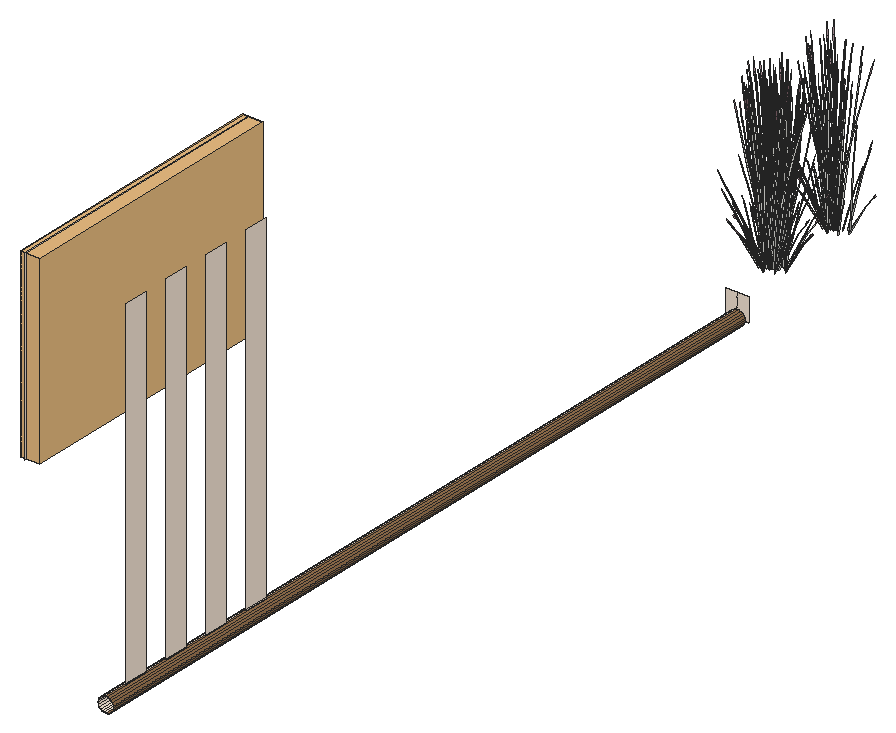
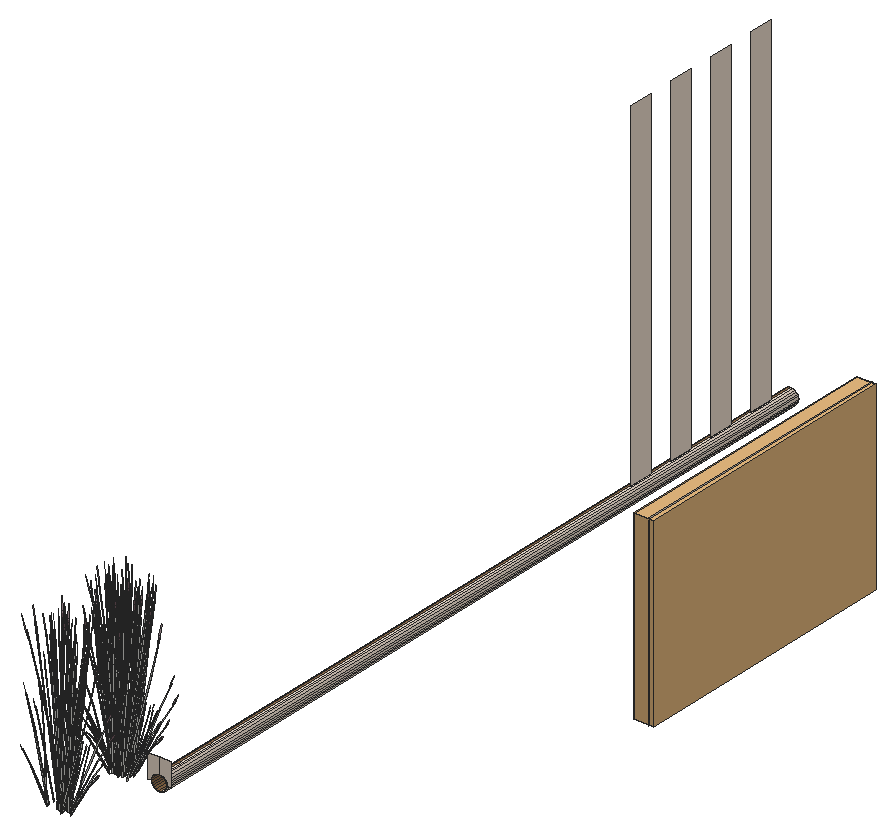
# SketchUp Ruby script. Lengths in inches.
U = 1.inch
M = Sketchup.active_model
def pt(a) = Geom::Point3d.new(a.map { |v| v * U })
def face(e, loops, mat)
  f = e.add_face(loops[0].map { |a| pt(a) })
  loops[1..].each { |l| e.add_face(l.map { |a| pt(a) }).erase! }
  f.material = f.back_material = mat if mat
  f
end
# faces: each face lists its corners as indices into pts; further lists are holes
def faces(e, pts, list, mat = nil) = list.each { |f| face(e, (f[0].is_a?(Array) ? f : [f]).map { |l| l.map { |i| pts[i] } }, mat) }
# xy, xz, yz: faces in a plane at the given z, y or x. An outline is a flat list of corners, or four numbers for a rectangle; further outlines are holes
def ring(l) = l.size == 4 ? [[l[0], l[1]], [l[2], l[1]], [l[2], l[3]], [l[0], l[3]]] : l.each_slice(2).to_a
def flat(e, list, mat, &to3) = list.each { |f| face(e, (f[0].is_a?(Array) ? f : [f]).map { |l| ring(l).map { |u, v| to3.(u, v) } }, mat) }
def xy(e, z, list, mat = nil) = flat(e, list, mat) { |x, y| [x, y, z] }
def xz(e, y, list, mat = nil) = flat(e, list, mat) { |x, z| [x, y, z] }
def yz(e, x, list, mat = nil) = flat(e, list, mat) { |y, z| [x, y, z] }
def lines(e, pts, list) = list.each { |a, b| e.add_line(pt(pts[a]), pt(pts[b])) }
# prism: a flat outline (further loops are holes) pulled along v
def prism(e, loops, v, mat = nil)
  f = face(e, loops, mat); d = Geom::Vector3d.new(v.map { |x| x * U })
  f.pushpull(f.normal.samedirection?(d) ? d.length : -d.length)
end
def box(e, o, s, mat = nil) = prism(e, [[o, [o[0] + s[0], o[1], o[2]], [o[0] + s[0], o[1] + s[1], o[2]], [o[0], o[1] + s[1], o[2]]]], [0, 0, s[2]], mat)
def at(x, y, z, deg = 0) = Geom::Transformation.translation(pt([x, y, z])) * Geom::Transformation.rotation(ORIGIN, Z_AXIS, deg.degrees)
def axes(o, x, y, z) = Geom::Transformation.new([*x, 0, *y, 0, *z, 0, *pt(o).to_a, 1])
def part(name) = M.definitions.add(name)
# library, detail: a bought-in or finely detailed component or shape, given as its bounding box
def library(name, o, s) = part(name).tap { |d| box(d.entities, o, s) }
def detail(e, o, s) = box(e.add_group.entities, o, s)
def put(e, d, t, mat = nil) = e.add_instance(d, t).tap { |i| i.material = mat if mat }
def group(e, t, mat = nil) = e.add_group.tap { |g| g.transformation = t; g.material = mat if mat }.entities
root = M.entities
M.materials.add("C01_Vanilla_Cream").color = [244, 228, 212]
M.materials.add("LightPink_Translucent").color = [144, 107, 117]
M.materials["LightPink_Translucent"].alpha = 0.75
M.materials.add("Wood_Floor_01_1K").color = [146, 111, 76]
c1 = library("Double casement window",[0,0,0],[5.02,56.42,60])
c2 = part("blade")
p = [[2.15,0.21,22],[0,0.17,0],[0.09,0.45,0],[2.18,0.31,22],[2.29,0.31,22],[0.38,0.45,0],
  [2.48,0.24,33],[2.49,0.24,33],[2.48,0.22,33]]
faces(c2.entities,p,[[0,1,2,3],[4,5,2,3],[6,3,4,7],[8,0,3,6]])
c3 = part("seeds")
p = [[0.3,-0.1,1.38],[-0.01,-0.03,1.59],[-0.01,-0.03,0.03],[0.14,-0.07,-0.07],[0.29,-0.03,3],[0.15,0.01,3.11]]
faces(c3.entities,p,[[0,1,2,3],[1,0,4,5]],"LightPink_Translucent")
c4 = part("blade with seeds")
put(c4.entities,c2,at(0,0,0))
put(c4.entities,c3,axes([2.4,0.25,30.99],[1.5799,-0.05474,1.17369],[-0.12525,1.92788,0.29478],[-0.07173,-0.02425,1.56792]))
xz(root,216,[[354,342,355,342,355.07,342.52,355.27,343,355.59,343.41,356,343.73,356.48,343.93,357,344,357,348,354,348],[359,342,360,342,360,348,357,348,357,344,357.52,343.93,358,343.73,358.41,343.41,358.73,343,358.93,342.52]],"C01_Vanilla_Cream")
yz(root,288,[[[72,348,144,396],[109.5,351,141,393],[75,351,106.5,393]]],"C01_Vanilla_Cream")
yz(root,357,[[18.46,340,24.91,344],[31.37,340,37.83,344],[44.28,340,50.74,344],[57.2,340,63.65,344],[18.46,344,24.91,432],
  [31.37,344,37.83,432],[44.28,344,50.74,432],[57.2,344,63.65,432]],"C01_Vanilla_Cream")
p = [[356.48,216,340.07],[357,216,340],[357,63.65,340],[357,57.2,340],[357,50.74,340],[357,44.28,340],
  [357,37.83,340],[357,31.37,340],[357,24.91,340],[357,18.46,340],[357,12,340],[356.48,12,340.07],
  [357.52,216,340.07],[357.52,12,340.07],[356,216,340.27],[356,12,340.27],[358,216,340.27],[358,12,340.27],
  [355.59,216,340.59],[355.59,12,340.59],[358.41,216,340.59],[358.41,12,340.59],[355.27,216,341],[355.27,12,341],
  [358.73,216,341],[358.73,12,341],[355.07,216,341.48],[355.07,12,341.48],[358.93,216,341.48],[358.93,12,341.48],
  [355,216,342],[355,12,342],[359,216,342],[359,12,342],[355.07,216,342.52],[355.07,12,342.52],
  [358.93,216,342.52],[358.93,12,342.52],[355.27,216,343],[355.27,12,343],[358.73,216,343],[358.73,12,343],
  [355.59,216,343.41],[355.59,12,343.41],[358.41,216,343.41],[358.41,12,343.41],[356,216,343.73],[356,12,343.73],
  [358,216,343.73],[358,12,343.73],[356.48,216,343.93],[356.48,12,343.93],[357.52,216,343.93],[357.52,12,343.93],
  [357,216,344],[357,12,344],[357,18.46,344],[357,24.91,344],[357,31.37,344],[357,37.83,344],
  [357,44.28,344],[357,50.74,344],[357,57.2,344],[357,63.65,344]]
faces(root,p,[[0,1,2,3,4,5,6,7,8,9,10,11],[14,0,11,15],[18,14,15,19],[22,18,19,23],[26,22,23,27],[30,26,27,31],[34,30,31,35],[38,34,35,39],
  [42,38,39,43],[46,42,43,47],[50,46,47,51],[54,50,51,55,56,57,58,59,60,61,62,63]],"C01_Vanilla_Cream")
faces(root,p,[[1,12,13,10,9,8,7,6,5,4,3,2],[12,16,17,13],[16,20,21,17],[20,24,25,21],[24,28,29,25],[28,32,33,29],[32,36,37,33],[36,40,41,37],
  [40,44,45,41],[44,48,49,45],[48,52,53,49],[52,54,63,62,61,60,59,58,57,56,55,53]],"Wood_Floor_01_1K")
put(root,c1,axes([286.7,72.24,348.3],[1,0,0],[0,1.27666,0],[0,0,0.79394]))
put(root,c4,axes([358.54,224.77,349.94],[-0.15825,0.09972,1.07251],[-0.47395,-0.17454,-0.23066],[0.08785,-0.21706,0.45856]))
put(root,c4,axes([356.09,224.58,349.94],[-0.03371,0.16116,1.07251],[-0.49286,0.13491,-0.23066],[-0.11521,-0.20831,0.45856]))
put(root,c4,axes([357.36,224.23,349.12],[-0.09338,0.01775,1.32257],[-0.51641,-0.1998,-0.20205],[0.00867,-0.16666,0.22528]))
put(root,c4,axes([357.95,223.98,350.07],[0.07142,0.28728,0.86145],[-0.3962,-0.15911,0.63294],[0.04263,-0.1471,0.18974]))
put(root,c4,axes([355.92,224.32,350.07],[0.29042,0.17147,0.86145],[-0.42295,0.10307,0.63294],[-0.0905,-0.13178,0.18974]))
put(root,c4,axes([355.6875,224.84,349.12],[-0.05393,0.0649,1.32257],[-0.545,0.13993,-0.20205],[-0.13166,-0.12729,0.22528]))
put(root,c4,axes([356.59,226.62,349.57],[-0.22864,-0.5052,-0.52377],[0.65862,-0.18195,-0.13747],[-0.02527,-0.17107,1.15612]))
put(root,c4,axes([359.64,225.08,349.12],[-0.08333,-0.03881,1.32257],[-0.21404,-0.4336,-0.20205],[0.14439,-0.11767,0.22528]))
put(root,c4,axes([356.5,225.17,349.78],[-0.34808,-0.49367,0],[0.58235,-0.27531,-0.38706],[0.13264,-0.0627,1.22783]))
put(root,c4,axes([357.26,224.57,349.6],[-0.38473,0.28263,-0.02919],[-0.35252,-0.30954,-0.13237],[-0.02482,-0.08771,0.43661]))
put(root,c4,axes([355.24,226.55,349.51],[0,-0.49266,-0.37238],[0.62289,0,0],[0,-0.11221,1.18128]))
put(root,c4,axes([356.97,225.09,349.51],[0.52105,-0.24633,-0.37238],[0.31144,0.44171,0],[0.11867,-0.0561,1.18128]))
put(root,c4,axes([360.0625,225.94,349.94],[-0.19889,-0.01459,1.07251],[-0.20376,-0.39145,-0.23066],[0.24434,-0.11074,0.45856]))
put(root,c4,axes([357.59,226.1,349.54],[0.375,-0.3703,-0.46765],[0.46584,0.33578,-0.12274],[0.15027,-0.09237,1.03225]))
put(root,c4,axes([360.29,225.22,350.07],[-0.18544,0.25079,0.86145],[-0.15939,-0.33694,0.63294],[0.15316,-0.08443,0.18974]))
put(root,c4,axes([356.93,226.75,349.66],[0.27012,-0.44393,-0.33554],[0.56127,0.21365,0.16149],[0,-0.10233,1.07733]))
put(root,c4,axes([357.18,226.53,350],[-0.06488,-0.56215,-0.21822],[0.6757,-0.03399,-0.37502],[0.11898,-0.07488,1.19781]))
put(root,c4,axes([355.51,226.5625,349.52],[0.38863,-0.30738,-0.23233],[0.38863,0.30738,0.23233],[0,-0.09901,1.0423]))
put(root,c4,axes([355.35,225.09,349.6],[-0.1606,0.40228,-0.02919],[-0.4943,-0.12375,-0.13237],[-0.07505,-0.0658,0.43661]))
put(root,c4,axes([356.87,227.12,350],[-0.62699,-0.23507,-0.21822],[0.3019,-0.49615,-0.37502],[-0.0197,-0.12182,1.19781]))
put(root,c4,axes([355.08,226.92,349.78],[-0.69617,0,0],[0,-0.55062,-0.38706],[0,-0.12541,1.22783]))
put(root,c4,axes([355.2,225.94,349.94],[0.1087,0.13716,1.07251],[-0.25048,0.37284,-0.23066],[-0.25719,-0.08912,0.45856]))
put(root,c4,axes([357.09,225.29,349.52],[0.51941,0.1219,-0.23233],[-0.13078,0.42928,0.23233],[0.10471,-0.0495,1.0423]))
put(root,c4,axes([355.625,226.78,349.75],[-0.51786,0.4142,0.23067],[-0.51817,-0.40984,-0.27369],[-0.01808,-0.11762,1.23664]))
put(root,c4,axes([357.27,226.97,349.82],[0.6273,0.23878,0.18048],[-0.3019,0.49615,0.37502],[0,-0.11437,1.20407]))
put(root,c4,axes([357.03,227.64,349.83],[0.14756,-0.58378,-0.17572],[0.69966,0.10176,0.38453],[-0.12225,-0.08062,1.1733]))
put(root,c4,axes([354.56,226.35,350.07],[0.35544,-0.03525,0.86145],[-0.22547,0.31061,0.63294],[-0.17565,-0.04659,0.18974]))
put(root,c4,axes([357.07,226.64,350.04],[-0.60457,0.03041,0.33554],[-0.05467,-0.50484,-0.16149],[0.10823,-0.05117,1.07733]))
put(root,c4,axes([355.51,227.01,349.86],[0,0.49266,0.37238],[-0.62289,0,0],[0,-0.11221,1.18128]))
put(root,c4,axes([359.0625,225.29,349.78],[0.34808,-0.49367,0],[0.58235,0.27531,-0.38706],[0.13264,0.0627,1.22783]))
put(root,c4,axes([356.98,227.4,349.66],[-0.33445,-0.41351,-0.33554],[0.50659,-0.29119,0.16149],[-0.10823,-0.05117,1.07733]))
put(root,c4,axes([357.05,226.82,349.77],[0.24206,0.5509,0.34316],[-0.69162,0.19157,0.13466],[0.00845,-0.10123,1.19142]))
put(root,c4,axes([360.43,227.24,349.49],[-0.35858,0.05912,1.06187],[-0.05708,-0.47061,0.06078],[0.25115,-0.07123,0.60425]))
put(root,c4,axes([361.08,226.83,349.7],[-0.34516,-0.31503,-0.04866],[0.37803,-0.28865,-0.22062],[0.10711,-0.02032,0.72768]))
put(root,c4,axes([356.92,227.25,350.04],[-0.27012,0.44393,0.33554],[-0.56127,-0.21365,-0.16149],[0,-0.10233,1.07733]))
put(root,c4,axes([357.92,226.87,349.65],[0,-0.57005,0],[0.69617,0,0],[0,0,1.34592]))
put(root,c4,axes([358.76,225.55,349.86],[-0.52105,-0.24633,0.37238],[0.31144,-0.44171,0],[0.11867,0.0561,1.18128]))
put(root,c4,axes([356.68,227.5625,349.54],[-0.57914,-0.08077,-0.46765],[0.12221,-0.49823,-0.12274],[-0.17283,-0.06037,1.03225]))
put(root,c4,axes([357.59,226.51,349.77],[-0.46162,0.4471,0.34316],[-0.54842,-0.39467,0.13466],[0.11129,-0.04462,1.19142]))
put(root,c4,axes([358.09,227.31,349.72],[-0.51786,-0.42404,-0.04598],[0.51817,-0.4243,0],[-0.01808,-0.01481,1.31678]))
put(root,c4,axes([356.79,225.77,349.86],[-0.16083,0.48962,0.13232],[-0.58854,-0.13856,0.26315],[0.10167,-0.00238,1.20305]))
put(root,c4,axes([356.54,226.17,349.2],[-0.548,0.19724,0.96696],[-0.17442,-0.56594,0.37572],[0.3365,0.00941,1.09981]))
put(root,c4,axes([358.01,226.32,349.96],[0.1074,-0.43968,0.1086],[0.52474,0.07632,-0.3101],[0.0955,0.04515,0.95058]))
put(root,c4,axes([357.11,227.36,349.77],[0.70367,0.1038,0.34316],[-0.1432,0.58624,0.13466],[-0.10283,-0.05661,1.19142]))
put(root,c4,axes([360.82,226.9375,349.12],[-0.0291,-0.0748,1.32257],[0.20181,-0.43752,-0.20205],[0.20357,-0.00629,0.22528]))
put(root,c4,axes([354.81,226.86,349.12],[0.01412,0.07764,1.32257],[-0.28464,0.40547,-0.20205],[-0.20218,-0.02044,0.22528]))
put(root,c4,axes([357.79,226.43,350.04],[-0.33445,-0.41351,0.33554],[0.50659,-0.29119,-0.16149],[0.10823,0.05117,1.07733]))
put(root,c4,axes([356.0625,228.32,349.52],[-0.13078,-0.42928,-0.23233],[0.51941,-0.1219,0.23233],[-0.10471,-0.0495,1.0423]))
put(root,c4,axes([356.73,228.3,349.86],[0.59825,-0.13076,0.13232],[0.14773,0.48663,0.26315],[-0.05336,-0.0709,1.20305]))
put(root,c4,axes([357.96,226.46,350],[0.56211,-0.32708,-0.21822],[0.3738,0.46216,-0.37502],[0.13869,0.04694,1.19781]))
put(root,c4,axes([355.92,228.51,349.51],[-0.52105,-0.24633,-0.37238],[0.31144,-0.44171,0],[-0.11867,-0.0561,1.18128]))
put(root,c4,axes([359.38,225.59,349.51],[0.52105,0.24633,-0.37238],[-0.31144,0.44171,0],[0.11867,0.0561,1.18128]))
put(root,c4,axes([358.39,227,349.65],[0.62289,0,0],[0,0.51004,0],[0,0,1.33805]))
put(root,c4,axes([357.33,227.64,350],[-0.56211,0.32708,-0.21822],[-0.3738,-0.46216,-0.37502],[-0.13869,-0.04694,1.19781]))
put(root,c4,axes([358.57,225.8,349.86],[-0.59825,0.13076,0.13232],[-0.14773,-0.48663,0.26315],[0.05336,0.0709,1.20305]))
put(root,c4,axes([359.23,225.77,349.52],[0.13078,0.42928,-0.23233],[-0.51941,0.1219,0.23233],[0.10471,0.0495,1.0423]))
put(root,c4,axes([358.1875,226.74,349.79],[-0.70367,-0.1038,0.36899],[0.1432,-0.58624,0.1448],[0.10283,0.05661,1.2811]))
put(root,c4,axes([357.625,228.18,349.65],[-0.18165,-0.42474,0],[0.51872,-0.14874,0],[0,0,1.15778]))
put(root,c4,axes([357.28,227.78,349.96],[-0.1074,0.43968,0.1086],[-0.52474,-0.07632,-0.3101],[-0.0955,-0.04515,0.95058]))
put(root,c4,axes([358.31,228.125,349.64],[0.5845,-0.16716,-0.14398],[0.20539,0.48152,0.00006],[0.06452,-0.01848,1.30423]))
put(root,c4,axes([358.51,228.32,349.86],[0.16083,-0.48962,0.13232],[0.58854,0.13856,0.26315],[-0.10167,0.00238,1.20305]))
put(root,c4,axes([358.375,227.21,349.66],[0.38863,0.31822,0],[-0.38863,0.31822,0],[0,0,1.2695]))
put(root,c4,axes([359.43,227.07,349.86],[-0.43742,-0.35886,0.13232],[0.44081,-0.34807,0.26315],[-0.04831,0.07329,1.20305]))
put(root,c4,axes([358.62,226.53,349.54],[0.57914,0.08077,-0.46765],[-0.12221,0.49823,-0.12274],[0.17283,0.06037,1.03225]))
put(root,c4,axes([361.18,227.4,350.07],[-0.34399,0.08133,0.86145],[0.16192,-0.33614,0.63294],[0.18249,0.023,0.18974]))
put(root,c4,axes([357.5,228.375,349.65],[-0.56127,-0.22118,0],[0.27012,-0.45959,0],[0,0,1.2203]))
put(root,c4,axes([357.96,227.79,349.85],[-0.54364,-0.39653,-0.18894],[0.45745,-0.44527,0.41347],[-0.14639,0.04639,1.26162]))
put(root,c4,axes([356.53,228.55,349.86],[0.52105,0.24633,0.37238],[-0.31144,0.44171,0],[-0.11867,-0.0561,1.18128]))
put(root,c4,axes([358.37,226.84,350.04],[0.27012,-0.44393,0.33554],[0.56127,0.21365,-0.16149],[0,0.10233,1.07733]))
put(root,c4,axes([358.27,227.1,349.72],[0,0.56976,-0.04228],[-0.69617,0,0],[0,0.01791,1.34526]))
put(root,c4,axes([358.32,226.69,349.66],[0.33445,0.41351,-0.33554],[-0.50659,0.29119,0.16149],[0.10823,0.05117,1.07733]))
put(root,c4,axes([356.23,228.8,349.78],[-0.34808,0.49367,0],[-0.58235,-0.27531,-0.38706],[-0.13264,-0.0627,1.22783]))
put(root,c4,axes([359.79,227.09,349.86],[0,-0.49266,0.37238],[0.62289,0,0],[0,0.11221,1.18128]))
put(root,c4,axes([358.23,227.46,350.04],[0.60457,-0.03041,0.33554],[0.05467,0.50484,-0.16149],[-0.10823,0.05117,1.07733]))
put(root,c4,axes([358.6,226.94,349.96],[0.51872,-0.14368,0.1086],[0.18165,0.41027,-0.3101],[0,0.09029,0.95058]))
put(root,c4,axes([357.6875,227.7,349.66],[-0.60457,0.03041,-0.33554],[-0.05467,-0.50484,0.16149],[-0.10823,0.05117,1.07733]))
put(root,c4,axes([360.53,227.94,349.94],[-0.13408,-0.12117,1.07251],[0.17446,-0.40083,-0.23066],[0.27128,0.0543,0.45856]))
put(root,c4,axes([358.14,228.38,349.65],[0.56127,0.22118,0],[-0.27012,0.45959,0],[0,0,1.31215]))
put(root,c4,axes([358.36,228.87,349.64],[-0.34375,-0.4954,-0.03857],[0.58235,-0.27531,0.38706],[-0.1435,0.04717,1.22723]))
put(root,c4,axes([358.24,227.67,349.96],[0.41131,0.296,0.1086],[-0.34309,0.33395,-0.3101],[-0.0955,0.04515,0.95058]))
put(root,c4,axes([358.67,228.59,349.86],[0.52105,-0.24633,0.37238],[0.31144,0.44171,0],[-0.11867,0.0561,1.18128]))
put(root,c4,axes([357.93,228.2,349.72],[0.24206,0.56598,-0.04509],[-0.69162,0.19832,0],[0.00845,0.01976,1.2913]))
put(root,c4,axes([358.2,228.81,349.52],[-0.51941,-0.1219,-0.23233],[0.13078,-0.42928,0.23233],[-0.10471,0.0495,1.0423]))
put(root,c4,axes([354.45,227.9375,349.94],[0.19348,0.04044,1.07251],[0.1247,0.41309,-0.23066],[-0.26282,0.07733,0.45856]))
put(root,c4,axes([360.21,227.17,349.78],[0.69617,0,0],[0,0.55062,-0.38706],[0,0.12541,1.22783]))
put(root,c4,axes([359.93,227.46,349.65],[-0.69582,-0.00394,-0.03732],[0,-0.55062,0.37457],[-0.02187,0.12535,1.18764]))
put(root,c4,axes([358.43,226.98,350],[0.62699,0.23507,-0.21822],[-0.3019,0.49615,-0.37502],[0.0197,0.12182,1.19781]))
put(root,c4,axes([354.05,228.8,350.07],[0.23202,-0.22328,0.86145],[0.09155,0.35348,0.63294],[-0.16768,0.06329,0.18974]))
put(root,c4,axes([359.79,227.54,349.52],[-0.38863,0.30738,-0.23233],[-0.38863,-0.30738,0.23233],[0,0.09901,1.0423]))
put(root,c4,axes([358.11,227.57,350],[0.06488,0.56215,-0.21822],[-0.6757,0.03399,-0.37502],[-0.11898,0.07488,1.19781]))
put(root,c4,axes([358.36,227.35,349.66],[-0.27012,0.44393,-0.33554],[-0.56127,-0.21365,0.16149],[0,0.10233,1.07733]))
put(root,c4,axes([357.71,227.99,349.54],[-0.375,0.3703,-0.46765],[-0.46584,-0.33578,-0.12274],[-0.15027,0.09237,1.03225]))
put(root,c4,axes([358.375,228.62,349.75],[0.697,0.16013,0.23067],[-0.17437,0.57237,-0.27369],[-0.11536,0.07164,1.23664]))
put(root,c4,axes([358.32,229,349.51],[-0.52105,0.24633,-0.37238],[-0.31144,-0.44171,0],[-0.11867,0.0561,1.18128]))
put(root,c4,axes([360.06,227.55,349.51],[0,0.49266,-0.37238],[-0.62289,0,0],[0,0.11221,1.18128]))
put(root,c4,axes([359.26,228.57,350.07],[-0.31347,-0.14166,0.86145],[0.40476,-0.14393,0.63294],[0.10917,0.12192,0.18974]))
put(root,c4,axes([358.8,228.93,349.78],[0.34808,0.49367,0],[-0.58235,0.27531,-0.38706],[-0.13264,0.0627,1.22783]))
put(root,c4,axes([359.35,229.09,349.12],[0.04056,-0.07113,1.32257],[0.51066,-0.20948,-0.20205],[0.15482,0.10842,0.22528]))
put(root,c4,axes([358.68,227.48,349.57],[0.20414,0.45107,-0.51909],[-0.58805,0.16245,-0.13624],[0.02256,0.15274,1.1458]))
put(root,c4,axes([354.66,229.03,349.12],[0.07468,0.04922,1.32257],[0.12663,0.45605,-0.20205],[-0.16551,0.09725,0.22528]))
put(root,c4,axes([359.3125,229.21,350],[-0.35702,-0.01545,0.78795],[0.23577,-0.32816,0.43504],[0.14104,0.11659,0.61808]))
put(root,c4,axes([358.15,228.42,349.94],[0.00982,-0.16331,1.07251],[0.4695,-0.18242,-0.23066],[0.14493,0.19547,0.45856]))
put(root,c4,axes([356.02,229.78,350.07],[-0.01441,-0.29294,0.86145],[0.36003,0.20894,0.63294],[-0.07081,0.13963,0.18974]))
put(root,c4,axes([356.97,229.08,349.12],[0.0901,-0.02681,1.32257],[0.54199,0.14755,-0.20205],[0.01585,0.1663,0.22528]))
put(root,c4,axes([355.72,229.15,350.12],[0.50577,-0.08724,0.04881],[0.11627,0.35148,-0.64728],[-0.03206,0.17792,0.5802]))
put(root,c4,axes([355.6,229.52,349.94],[0.17569,-0.07772,1.07251],[0.43377,0.23434,-0.23066],[-0.12911,0.20277,0.45856]))
put(root,c4,axes([358.54,245.34,349.94],[-0.15825,0.09972,1.07251],[-0.47395,-0.17454,-0.23066],[0.08785,-0.21706,0.45856]))
put(root,c4,axes([356.09,245.15,349.94],[-0.03371,0.16116,1.07251],[-0.49286,0.13491,-0.23066],[-0.11521,-0.20831,0.45856]))
put(root,c4,axes([357.36,244.8,349.12],[-0.09338,0.01775,1.32257],[-0.51641,-0.1998,-0.20205],[0.00867,-0.16666,0.22528]))
put(root,c4,axes([355.6875,245.41,349.12],[-0.05393,0.0649,1.32257],[-0.545,0.13993,-0.20205],[-0.13166,-0.12729,0.22528]))
put(root,c4,axes([356.59,247.19,349.57],[-0.22864,-0.5052,-0.52377],[0.65862,-0.18195,-0.13747],[-0.02527,-0.17107,1.15612]))
put(root,c4,axes([359.64,245.65,349.12],[-0.08333,-0.03881,1.32257],[-0.21404,-0.4336,-0.20205],[0.14439,-0.11767,0.22528]))
put(root,c4,axes([356.5,245.74,349.78],[-0.34808,-0.49367,0],[0.58235,-0.27531,-0.38706],[0.13264,-0.0627,1.22783]))
put(root,c4,axes([357.26,245.15,349.6],[-0.38473,0.28263,-0.02919],[-0.35252,-0.30954,-0.13237],[-0.02482,-0.08771,0.43661]))
put(root,c4,axes([355.24,247.125,349.51],[0,-0.49266,-0.37238],[0.62289,0,0],[0,-0.11221,1.18128]))
put(root,c4,axes([356.97,245.67,349.51],[0.52105,-0.24633,-0.37238],[0.31144,0.44171,0],[0.11867,-0.0561,1.18128]))
put(root,c4,axes([360.0625,246.52,349.94],[-0.19889,-0.01459,1.07251],[-0.20376,-0.39145,-0.23066],[0.24434,-0.11074,0.45856]))
put(root,c4,axes([357.59,246.68,349.54],[0.375,-0.3703,-0.46765],[0.46584,0.33578,-0.12274],[0.15027,-0.09237,1.03225]))
put(root,c4,axes([356.93,247.33,349.66],[0.27012,-0.44393,-0.33554],[0.56127,0.21365,0.16149],[0,-0.10233,1.07733]))
put(root,c4,axes([357.18,247.11,350],[-0.06488,-0.56215,-0.21822],[0.6757,-0.03399,-0.37502],[0.11898,-0.07488,1.19781]))
put(root,c4,axes([355.51,247.13,349.52],[0.38863,-0.30738,-0.23233],[0.38863,0.30738,0.23233],[0,-0.09901,1.0423]))
put(root,c4,axes([355.35,245.66,349.6],[-0.1606,0.40228,-0.02919],[-0.4943,-0.12375,-0.13237],[-0.07505,-0.0658,0.43661]))
put(root,c4,axes([356.87,247.69,350],[-0.62699,-0.23507,-0.21822],[0.3019,-0.49615,-0.37502],[-0.0197,-0.12182,1.19781]))
put(root,c4,axes([355.08,247.5,349.78],[-0.69617,0,0],[0,-0.55062,-0.38706],[0,-0.12541,1.22783]))
put(root,c4,axes([355.2,246.51,349.94],[0.1087,0.13716,1.07251],[-0.25048,0.37284,-0.23066],[-0.25719,-0.08912,0.45856]))
put(root,c4,axes([357.09,245.86,349.52],[0.51941,0.1219,-0.23233],[-0.13078,0.42928,0.23233],[0.10471,-0.0495,1.0423]))
put(root,c4,axes([355.625,247.35,349.75],[-0.51786,0.4142,0.23067],[-0.51817,-0.40984,-0.27369],[-0.01808,-0.11762,1.23664]))
put(root,c4,axes([357.27,247.55,349.82],[0.6273,0.23878,0.18048],[-0.3019,0.49615,0.37502],[0,-0.11437,1.20407]))
put(root,c4,axes([357.03,248.22,349.83],[0.14756,-0.58378,-0.17572],[0.69966,0.10176,0.38453],[-0.12225,-0.08062,1.1733]))
put(root,c4,axes([354.56,246.93,350.07],[0.35544,-0.03525,0.86145],[-0.22547,0.31061,0.63294],[-0.17565,-0.04659,0.18974]))
put(root,c4,axes([357.07,247.21,350.04],[-0.60457,0.03041,0.33554],[-0.05467,-0.50484,-0.16149],[0.10823,-0.05117,1.07733]))
put(root,c4,axes([355.51,247.58,349.86],[0,0.49266,0.37238],[-0.62289,0,0],[0,-0.11221,1.18128]))
put(root,c4,axes([359.0625,245.87,349.78],[0.34808,-0.49367,0],[0.58235,0.27531,-0.38706],[0.13264,0.0627,1.22783]))
put(root,c4,axes([356.98,247.98,349.66],[-0.33445,-0.41351,-0.33554],[0.50659,-0.29119,0.16149],[-0.10823,-0.05117,1.07733]))
put(root,c4,axes([357.05,247.4,349.77],[0.24206,0.5509,0.34316],[-0.69162,0.19157,0.13466],[0.00845,-0.10123,1.19142]))
put(root,c4,axes([360.43,247.82,349.49],[-0.35858,0.05912,1.06187],[-0.05708,-0.47061,0.06078],[0.25115,-0.07123,0.60425]))
put(root,c4,axes([361.08,247.4,349.7],[-0.34516,-0.31503,-0.04866],[0.37803,-0.28865,-0.22062],[0.10711,-0.02032,0.72768]))
put(root,c4,axes([356.92,247.83,350.04],[-0.27012,0.44393,0.33554],[-0.56127,-0.21365,-0.16149],[0,-0.10233,1.07733]))
put(root,c4,axes([357.92,247.44,349.65],[0,-0.57005,0],[0.69617,0,0],[0,0,1.34592]))
put(root,c4,axes([358.76,246.125,349.86],[-0.52105,-0.24633,0.37238],[0.31144,-0.44171,0],[0.11867,0.0561,1.18128]))
put(root,c4,axes([356.68,248.14,349.54],[-0.57914,-0.08077,-0.46765],[0.12221,-0.49823,-0.12274],[-0.17283,-0.06037,1.03225]))
put(root,c4,axes([357.59,247.08,349.77],[-0.46162,0.4471,0.34316],[-0.54842,-0.39467,0.13466],[0.11129,-0.04462,1.19142]))
put(root,c4,axes([358.09,247.88,349.72],[-0.51786,-0.42404,-0.04598],[0.51817,-0.4243,0],[-0.01808,-0.01481,1.31678]))
put(root,c4,axes([356.79,246.35,349.86],[-0.16083,0.48962,0.13232],[-0.58854,-0.13856,0.26315],[0.10167,-0.00238,1.20305]))
put(root,c4,axes([356.54,246.74,349.2],[-0.548,0.19724,0.96696],[-0.17442,-0.56594,0.37572],[0.3365,0.00941,1.09981]))
put(root,c4,axes([358.01,246.89,349.96],[0.1074,-0.43968,0.1086],[0.52474,0.07632,-0.3101],[0.0955,0.04515,0.95058]))
put(root,c4,axes([357.11,247.93,349.77],[0.70367,0.1038,0.34316],[-0.1432,0.58624,0.13466],[-0.10283,-0.05661,1.19142]))
put(root,c4,axes([360.82,247.51,349.12],[-0.0291,-0.0748,1.32257],[0.20181,-0.43752,-0.20205],[0.20357,-0.00629,0.22528]))
put(root,c4,axes([354.81,247.43,349.12],[0.01412,0.07764,1.32257],[-0.28464,0.40547,-0.20205],[-0.20218,-0.02044,0.22528]))
put(root,c4,axes([357.79,247.01,350.04],[-0.33445,-0.41351,0.33554],[0.50659,-0.29119,-0.16149],[0.10823,0.05117,1.07733]))
put(root,c4,axes([356.0625,248.9,349.52],[-0.13078,-0.42928,-0.23233],[0.51941,-0.1219,0.23233],[-0.10471,-0.0495,1.0423]))
